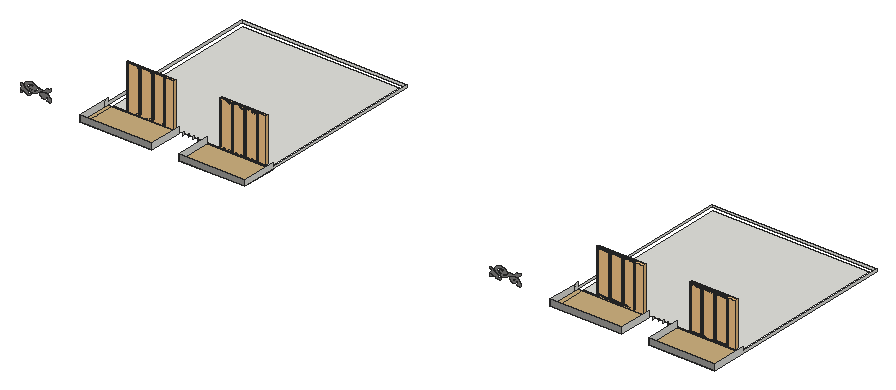
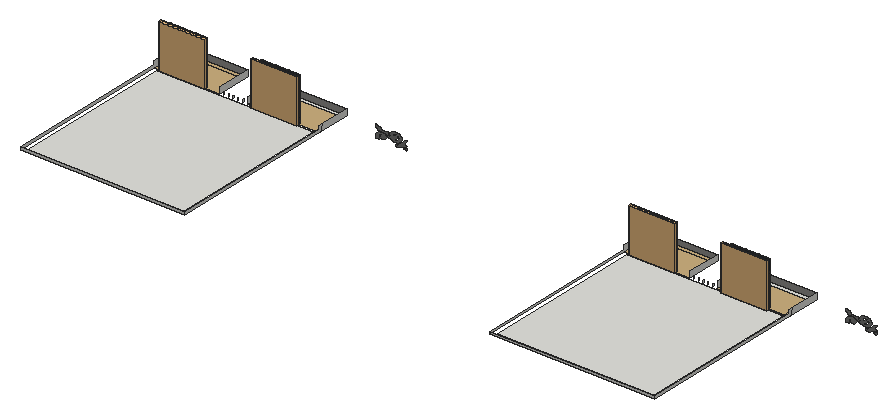
# SketchUp Ruby script. Lengths in inches.
U = 1.inch
M = Sketchup.active_model
def pt(a) = Geom::Point3d.new(a.map { |v| v * U })
def face(e, loops, mat)
  f = e.add_face(loops[0].map { |a| pt(a) })
  loops[1..].each { |l| e.add_face(l.map { |a| pt(a) }).erase! }
  f.material = f.back_material = mat if mat
  f
end
# faces: each face lists its corners as indices into pts; further lists are holes
def faces(e, pts, list, mat = nil) = list.each { |f| face(e, (f[0].is_a?(Array) ? f : [f]).map { |l| l.map { |i| pts[i] } }, mat) }
# xy, xz, yz: faces in a plane at the given z, y or x. An outline is a flat list of corners, or four numbers for a rectangle; further outlines are holes
def ring(l) = l.size == 4 ? [[l[0], l[1]], [l[2], l[1]], [l[2], l[3]], [l[0], l[3]]] : l.each_slice(2).to_a
def flat(e, list, mat, &to3) = list.each { |f| face(e, (f[0].is_a?(Array) ? f : [f]).map { |l| ring(l).map { |u, v| to3.(u, v) } }, mat) }
def xy(e, z, list, mat = nil) = flat(e, list, mat) { |x, y| [x, y, z] }
def xz(e, y, list, mat = nil) = flat(e, list, mat) { |x, z| [x, y, z] }
def yz(e, x, list, mat = nil) = flat(e, list, mat) { |y, z| [x, y, z] }
def lines(e, pts, list) = list.each { |a, b| e.add_line(pt(pts[a]), pt(pts[b])) }
# prism: a flat outline (further loops are holes) pulled along v
def prism(e, loops, v, mat = nil)
  f = face(e, loops, mat); d = Geom::Vector3d.new(v.map { |x| x * U })
  f.pushpull(f.normal.samedirection?(d) ? d.length : -d.length)
end
def box(e, o, s, mat = nil) = prism(e, [[o, [o[0] + s[0], o[1], o[2]], [o[0] + s[0], o[1] + s[1], o[2]], [o[0], o[1] + s[1], o[2]]]], [0, 0, s[2]], mat)
def at(x, y, z, deg = 0) = Geom::Transformation.translation(pt([x, y, z])) * Geom::Transformation.rotation(ORIGIN, Z_AXIS, deg.degrees)
def axes(o, x, y, z) = Geom::Transformation.new([*x, 0, *y, 0, *z, 0, *pt(o).to_a, 1])
def part(name) = M.definitions.add(name)
# library, detail: a bought-in or finely detailed component or shape, given as its bounding box
def library(name, o, s) = part(name).tap { |d| box(d.entities, o, s) }
def detail(e, o, s) = box(e.add_group.entities, o, s)
def put(e, d, t, mat = nil) = e.add_instance(d, t).tap { |i| i.material = mat if mat }
def group(e, t, mat = nil) = e.add_group.tap { |g| g.transformation = t; g.material = mat if mat }.entities
root = M.entities
M.materials.add("Wine2").color = [0, 0, 0]
M.materials["Wine2"].alpha = 0
M.materials.add("[0043_SaddleBrown]4").color = [124, 123, 122]
M.materials.add("[0130_Gainsboro]").color = [39, 45, 50]
M.materials.add("[Granite Light Gray]").color = [149, 148, 144]
M.materials.add("[Wood Floor Light]").color = [204, 176, 127]
c1 = part("Framed glazing panel")
xy(c1.entities,0,[[0,-0.98,43.07,0],[0,0,43.07,1.4]],"[0130_Gainsboro]")
xy(c1.entities,0.3,[[0.3,-1.43,42.77,-0.98]],"[0130_Gainsboro]")
xy(c1.entities,2.95,[[2.95,-1.43,40.12,-0.63],[2.95,-0.63,40.12,0],[2.95,0,40.12,0.64],[2.95,0.64,40.12,1.4]],"[0130_Gainsboro]")
xy(c1.entities,3.54,[[3.54,-0.63,39.53,0],[3.54,0,39.53,0.64]],"[0130_Gainsboro]")
xy(c1.entities,111.8125,[[3.54,-0.63,39.53,0],[3.54,0,39.53,0.64]],"[0130_Gainsboro]")
xy(c1.entities,112.4,[[2.95,-1.43,40.12,-0.63],[2.95,-0.63,40.12,0],[2.95,0,40.12,0.64],[2.95,0.64,40.12,1.4]],"[0130_Gainsboro]")
xy(c1.entities,115.05,[[0.3,-1.43,42.77,-0.98]],"[0130_Gainsboro]")
xy(c1.entities,115.35,[[0,-0.98,43.07,0],[0,0,43.07,1.4]],"[0130_Gainsboro]")
xz(c1.entities,-1.43,[[[0.3,0.3,42.77,115.05],[2.95,2.95,40.12,112.4]]],"[0130_Gainsboro]")
xz(c1.entities,-0.98,[[[0,0,43.07,115.35],[0.3,0.3,42.77,115.05]]],"[0130_Gainsboro]")
xz(c1.entities,-0.63,[[[2.95,2.95,40.12,112.4],[3.54,3.54,39.53,111.8125]]],"[0130_Gainsboro]")
xz(c1.entities,0,[[3.54,3.54,39.53,111.8125]],"Wine2")
xz(c1.entities,0,[[[0,0,43.07,115.35],[2.95,2.95,40.12,112.4]],[[2.95,2.95,40.12,112.4],[3.54,3.54,39.53,111.8125]]],"[0130_Gainsboro]")
xz(c1.entities,0.64,[[[2.95,2.95,40.12,112.4],[3.54,3.54,39.53,111.8125]]],"[0130_Gainsboro]")
xz(c1.entities,1.4,[[[0,0,43.07,115.35],[2.95,2.95,40.12,112.4]]],"[0130_Gainsboro]")
yz(c1.entities,0,[[-0.98,0,0,115.35],[0,0,1.4,115.35]],"[0130_Gainsboro]")
yz(c1.entities,0.3,[[-1.43,0.3,-0.98,115.05]],"[0130_Gainsboro]")
yz(c1.entities,2.95,[[-1.43,2.95,-0.63,112.4],[-0.63,2.95,0,112.4],[0,2.95,0.64,112.4],[0.64,2.95,1.4,112.4]],"[0130_Gainsboro]")
yz(c1.entities,3.54,[[-0.63,3.54,0,111.8125],[0,3.54,0.64,111.8125]],"[0130_Gainsboro]")
yz(c1.entities,39.53,[[-0.63,3.54,0,111.8125],[0,3.54,0.64,111.8125]],"[0130_Gainsboro]")
yz(c1.entities,40.12,[[-1.43,2.95,-0.63,112.4],[-0.63,2.95,0,112.4],[0,2.95,0.64,112.4],[0.64,2.95,1.4,112.4]],"[0130_Gainsboro]")
yz(c1.entities,42.77,[[-1.43,0.3,-0.98,115.05]],"[0130_Gainsboro]")
yz(c1.entities,43.07,[[-0.98,0,0,115.35],[0,0,1.4,115.35]],"[0130_Gainsboro]")
c2 = part("Glazing assembly")
put(c2.entities,c1,axes([90.57,1.43,0],[1.05148,0,0],[0,1,0],[0,0,1]))
put(c2.entities,c1,axes([0,1.43,0],[1.05148,0,0],[0,1,0],[0,0,1]))
put(c2.entities,c1,axes([45.29,1.43,0],[1.05148,0,0],[0,1,0],[0,0,1]))
c3 = library("Curtains",[0,0,0],[121.73,8.19,117.22])
xy(root,640.875,[[3103.26,651.03,3204.51,657.03],[3351.01,651.03,3452.26,657.03],[4353.89,651.03,4455.14,657.03],[4601.63,651.03,4702.88,657.03]])
xy(root,646.4375,[[3053.01,559.875,3243.69,570.83],[4303.63,559.875,4494.32,570.83],[3064.33,657.03,3480.11,1085.17],[4314.96,657.03,4730.74,1085.17]])
xy(root,646.4375,[[3316.14,559.875,3491.44,570.83],[4566.77,559.875,4742.06,570.83],[3053.01,570.83,3064.33,651.03],[3064.33,570.83,3243.69,651.03],[3316.14,570.83,3480.11,651.03],
  [3480.11,570.83,3491.44,651.03],[4303.63,570.83,4314.96,651.03],[4314.96,570.83,4494.32,651.03],[4566.77,570.83,4730.74,651.03],[4730.74,570.83,4742.06,651.03]],"[Wood Floor Light]")
xz(root,559.875,[[3053.01,646.4375,3243.69,662.4375],[3316.14,646.4375,3491.44,662.4375],[4303.63,646.4375,4494.32,662.4375],[4566.77,646.4375,4742.06,662.4375]],"[Granite Light Gray]")
xz(root,589.17,[[2869.93,640.49,2870.29,640.8,2870.68,641.09,2871.09,641.36,2871.54,641.62,2872.02,641.85,2872.52,642.07,2873.04,642.26,2873.59,642.43,2874.15,642.58,2874.73,642.71,2875.32,642.81,2875.92,642.89,2875.55,643.17,2875.15,643.4375,2874.72,643.68,2874.27,643.91,2873.79,644.125,2873.28,644.3125,2872.76,644.48,2872.22,644.62,2871.66,644.74,2871.1,644.83,2870.52,644.9,2869.93,644.94],[4120.56,640.49,4120.91,640.8,4121.3,641.09,4121.72,641.36,4122.17,641.62,4122.64,641.85,4123.15,642.07,4123.67,642.26,4124.21,642.43,4124.77,642.58,4125.35,642.71,4125.94,642.81,4126.54,642.89,4126.17,643.17,4125.78,643.4375,4125.35,643.68,4124.89,643.91,4124.41,644.125,4123.91,644.3125,4123.39,644.48,4122.85,644.62,4122.29,644.74,4121.72,644.83,4121.14,644.9,4120.56,644.94],[2893.58,641.03,2894.6,641.04,2895.41,641.12,2896.17,641.3125,2896.85,641.61,2897.4,641.99,2897.79,642.43,2898.01,642.92,2898.05,643.43,2897.9,643.93,2897.57,644.39,2897.08,644.8,2896.46,645.13,2895.73,645.37,2895.62,644.86,2895.3,644.38,2894.79,643.98,2894.125,643.66,2893.35,643.47,2892.52,643.4,2891.7,643.47,2890.92,643.66,2890.26,643.98,2889.75,644.38,2889.43,644.86,2889.32,645.37,2889.28,645.77,2889.25,646.18,2889.24,646.58,2889.25,646.99,2889.28,647.39,2889.32,647.8,2889.39,648.2,2889.47,648.6,2889.5625,649,2889.68,649.4,2889.8125,649.8,2889.96,650.19,2888.5,650.55,2887.09,650.99,2885.73,651.48,2884.45,652.05,2883.24,652.67,2882.12,653.35,2881.09,654.09,2880.16,654.87,2879.33,655.69,2878.62,656.56,2878.01,657.45,2877.52,658.375,2877,658.8,2876.45,659.22,2875.89,659.625,2875.3,660.02,2874.69,660.41,2874.06,660.78,2873.42,661.14,2872.76,661.49,2872.07,661.82,2871.375,662.14,2870.66,662.45,2869.93,662.74,2869.93,660.01,2870.95,659.23,2871.81,658.39,2872.49,657.48,2872.98,656.53,2873.28,655.56,2873.38,654.5625,2873.28,653.57,2872.98,652.59,2872.49,651.64,2871.81,650.74,2870.95,649.89,2869.93,649.12,2869.93,648.22,2871.22,648.05,2872.49,647.85,2873.74,647.6,2874.97,647.32,2876.18,647,2877.35,646.63,2878.49,646.23,2879.6,645.8,2880.67,645.33,2881.69,644.82,2882.67,644.28,2883.61,643.71,2884.34,643.28,2885.11,642.88,2885.94,642.51,2886.8,642.18,2887.7,641.89,2888.625,641.64,2889.58,641.43,2890.5625,641.26,2891.56,641.14,2892.57,641.0625],[4144.2,641.03,4145.22,641.04,4146.04,641.12,4146.8,641.3125,4147.47,641.61,4148.02,641.99,4148.42,642.43,4148.64,642.92,4148.68,643.43,4148.53,643.93,4148.2,644.39,4147.71,644.8,4147.08,645.13,4146.35,645.37,4146.24,644.86,4145.92,644.38,4145.41,643.98,4144.75,643.66,4143.98,643.47,4143.15,643.4,4142.32,643.47,4141.55,643.66,4140.88,643.98,4140.375,644.38,4140.06,644.86,4139.95,645.37,4139.9,645.77,4139.875,646.18,4139.87,646.58,4139.88,646.99,4139.9,647.39,4139.95,647.8,4140.01,648.2,4140.09,648.6,4140.1875,649,4140.3,649.4,4140.4375,649.8,4140.59,650.19,4139.125,650.55,4137.71,650.99,4136.36,651.48,4135.08,652.05,4133.87,652.67,4132.75,653.35,4131.72,654.09,4130.79,654.87,4129.96,655.69,4129.24,656.56,4128.64,657.45,4128.15,658.375,4127.625,658.8,4127.08,659.22,4126.51,659.625,4125.92,660.02,4125.32,660.41,4124.69,660.78,4124.04,661.14,4123.38,661.49,4122.7,661.82,4122,662.14,4121.29,662.45,4120.56,662.74,4120.56,660.01,4121.58,659.23,4122.43,658.39,4123.11,657.48,4123.61,656.53,4123.91,655.56,4124.01,654.5625,4123.91,653.57,4123.61,652.59,4123.11,651.64,4122.43,650.74,4121.58,649.89,4120.56,649.12,4120.56,648.22,4121.84,648.05,4123.12,647.85,4124.37,647.6,4125.6,647.32,4126.8,647,4127.98,646.63,4129.12,646.23,4130.22,645.8,4131.29,645.33,4132.32,644.82,4133.3,644.28,4134.23,643.71,4134.96,643.28,4135.74,642.88,4136.56,642.51,4137.42,642.18,4138.32,641.89,4139.25,641.64,4140.21,641.43,4141.1875,641.26,4142.18,641.14,4143.19,641.0625],[2950.32,642.71,2950.32,650.32,2949.96,650.87,2949.58,651.42,2949.18,651.96,2948.77,652.5,2948.35,653.03,2947.9,653.5625,2947.45,654.09,2946.97,654.61,2946.49,655.12,2945.99,655.63,2945.47,656.13,2944.94,656.63,2944.08,657.33,2943.1,657.96,2942,658.52,2940.8125,659,2939.54,659.39,2938.2,659.6875,2936.81,659.89,2935.39,659.99,2933.97,659.99,2932.56,659.89,2931.17,659.69,2929.83,659.39,2927.89,658.73,2926.2,657.86,2924.8125,656.81,2923.78,655.61,2923.15,654.31,2922.93,652.96,2923.15,651.61,2923.78,650.31,2924.8125,649.11,2926.2,648.05,2927.89,647.18,2929.83,646.53,2930.47,646.3,2931.16,646.13,2931.89,646.04,2932.63,646.01,2933.37,646.0625,2934.09,646.18,2934.77,646.37,2935.39,646.62,2935.93,646.93,2936.4,647.28,2936.76,647.68,2937.02,648.11,2937.38,648.49,2937.66,648.9,2937.83,649.33,2937.91,649.77,2937.88,650.21,2937.76,650.64,2937.54,651.0625,2937.22,651.46,2936.8125,651.82,2936.33,652.15,2935.77,652.43,2935.16,652.66,2934.8,652.54,2934.46,652.41,2934.13,652.27,2933.82,652.11,2933.53,651.94,2933.26,651.76,2933.01,651.57,2932.79,651.37,2932.58,651.15,2932.4,650.93,2932.25,650.71,2932.12,650.47,2931.35,650.76,2930.6875,651.12,2930.14,651.56,2929.74,652.05,2929.49,652.57,2929.41,653.12,2929.49,653.67,2929.74,654.19,2930.14,654.68,2930.6875,655.12,2931.35,655.48,2932.12,655.77,2933.05,655.79,2933.98,655.77,2934.91,655.7,2935.83,655.6,2936.73,655.45,2937.61,655.26,2938.47,655.03,2939.29,654.76,2940.09,654.46,2940.84,654.12,2941.55,653.75,2942.21,653.34,2942.79,652.56,2943.26,651.75,2943.61,650.91,2943.83,650.07,2943.93,649.21,2943.9,648.35,2943.75,647.49,2943.47,646.65,2943.07,645.82,2942.55,645.03,2941.92,644.26,2941.17,643.53,2941.93,643.69,2942.72,643.8125,2943.51,643.89,2944.32,643.93,2945.12,643.92,2945.92,643.87,2946.72,643.78,2947.49,643.64,2948.25,643.47,2948.97,643.25,2949.67,643],
  [4200.95,642.71,4200.95,650.32,4200.58,650.87,4200.2,651.42,4199.81,651.96,4199.4,652.5,4198.97,653.03,4198.53,653.5625,4198.07,654.09,4197.6,654.61,4197.11,655.12,4196.61,655.63,4196.1,656.13,4195.57,656.63,4194.71,657.33,4193.73,657.96,4192.63,658.52,4191.4375,659,4190.16,659.39,4188.82,659.6875,4187.43,659.89,4186.02,659.99,4184.6,659.99,4183.18,659.89,4181.79,659.69,4180.45,659.39,4178.52,658.73,4176.83,657.86,4175.4375,656.81,4174.41,655.61,4173.77,654.31,4173.56,652.96,4173.77,651.61,4174.41,650.31,4175.4375,649.11,4176.83,648.05,4178.52,647.18,4180.45,646.53,4181.1,646.3,4181.79,646.13,4182.51,646.04,4183.26,646.01,4184,646.0625,4184.71,646.18,4185.39,646.37,4186.01,646.62,4186.56,646.93,4187.02,647.28,4187.39,647.68,4187.64,648.11,4188.01,648.49,4188.28,648.9,4188.46,649.33,4188.53,649.77,4188.51,650.21,4188.38,650.64,4188.16,651.0625,4187.84,651.46,4187.4375,651.82,4186.95,652.15,4186.4,652.43,4185.78,652.66,4185.43,652.54,4185.09,652.41,4184.76,652.27,4184.45,652.11,4184.16,651.94,4183.89,651.76,4183.64,651.57,4183.41,651.37,4183.21,651.15,4183.03,650.93,4182.87,650.71,4182.74,650.47,4181.98,650.76,4181.3125,651.12,4180.77,651.56,4180.36,652.05,4180.12,652.57,4180.03,653.12,4180.12,653.67,4180.36,654.19,4180.77,654.68,4181.3125,655.12,4181.98,655.48,4182.74,655.77,4183.68,655.79,4184.61,655.77,4185.54,655.7,4186.45,655.6,4187.36,655.45,4188.24,655.26,4189.09,655.03,4189.92,654.76,4190.71,654.46,4191.46,654.12,4192.17,653.75,4192.83,653.34,4193.42,652.56,4193.89,651.75,4194.23,650.91,4194.46,650.07,4194.56,649.21,4194.53,648.35,4194.375,647.49,4194.1,646.65,4193.69,645.82,4193.17,645.03,4192.54,644.26,4191.8,643.53,4192.56,643.69,4193.34,643.8125,4194.14,643.89,4194.94,643.93,4195.75,643.92,4196.55,643.87,4197.34,643.78,4198.12,643.64,4198.87,643.47,4199.6,643.25,4200.29,643],[2900.61,650.01,2903.77,650.11,2906.85,650.55,2909.77,651.29,2912.44,652.33,2914.79,653.63,2916.75,655.16,2917.29,655.79,2917.88,656.41,2918.52,657.01,2919.2,657.59,2919.92,658.15,2920.69,658.6875,2921.5,659.2,2922.35,659.69,2923.23,660.16,2924.15,660.6,2925.1,661.01,2926.08,661.4,2927.38,661.78,2928.72,662.11,2930.08,662.4,2931.47,662.65,2932.875,662.84,2934.3,662.99,2935.73,663.09,2937.17,663.14,2938.61,663.14,2940.05,663.1,2941.48,663,2942.91,662.86,2943.46,663.4,2944.03,663.94,2944.61,664.48,2945.2,665.01,2945.8,665.54,2946.42,666.0625,2947.04,666.58,2948.32,667.6,2948.98,668.1,2949.65,668.59,2950.32,669.09,2950.32,674.83,2949.96,674.24,2949.46,673.68,2948.84,673.17,2948.11,672.72,2947.29,672.34,2946.38,672.04,2945.42,671.81,2944.41,671.67,2943.38,671.62,2942.35,671.65,2941.34,671.78,2940.37,671.99,2939.92,670.62,2939.11,669.32,2937.94,668.13,2936.47,667.08,2934.72,666.19,2932.75,665.51,2930.62,665.04,2928.38,664.8,2926.12,664.79,2923.89,665.03,2921.75,665.49,2919.78,666.17,2919.72,664.45,2919.25,662.75,2918.39,661.12,2917.14,659.57,2915.55,658.15,2913.64,656.89,2911.45,655.82,2909.04,654.95,2906.4375,654.3,2903.71,653.89,2900.92,653.73,2898.12,653.82,2895.67,654.4375,2893.45,655.33,2891.56,656.48,2890.07,657.82,2889.02,659.32,2888.47,660.91,2888.43,662.54,2888.89,664.14,2889.86,665.66,2891.28,667.03,2893.11,668.21,2895.27,669.15,2896.66,669.53,2898.16,669.73,2899.68,669.73,2901.18,669.55,2902.58,669.18,2903.83,668.64,2904.875,667.96,2905.67,667.16,2906.1875,666.28,2906.4,665.35,2906.3,664.42,2905.9,663.52,2905.62,663.1875,2905.24,662.89,2904.78,662.65,2904.25,662.48,2903.67,662.37,2903.06,662.33,2902.46,662.37,2901.88,662.48,2901.35,662.65,2900.89,662.89,2900.51,663.1875,2900.23,663.52,2900.09,663.71,2899.93,663.89,2899.75,664.07,2899.54,664.24,2899.31,664.39,2899.06,664.53,2898.79,664.66,2898.5,664.78,2898.2,664.88,2897.89,664.97,2897.57,665.04,2897.24,665.09,2896.66,664.88,2896.125,664.63,2895.64,664.34,2895.22,664.01,2894.87,663.66,2894.59,663.28,2894.39,662.89,2894.27,662.48,2894.23,662.07,2894.27,661.65,2894.4,661.25,2894.61,660.85,2895,660.32,2895.48,659.82,2896.04,659.36,2896.68,658.93,2897.4,658.55,2898.17,658.21,2899,657.94,2899.88,657.71,2900.79,657.55,2901.72,657.44,2902.66,657.4,2903.61,657.42,2905.1,657.57,2906.55,657.83,2907.92,658.22,2909.2,658.71,2910.37,659.3,2911.39,659.98,2912.26,660.74,2912.95,661.56,2913.46,662.4375,2913.78,663.35,2913.9,664.27,2913.81,665.2,2913.2,666.59,2912.28,667.91,2911.0625,669.15,2909.57,670.26,2907.84,671.23,2905.89,672.04,2903.79,672.67,2901.55,673.12,2899.24,673.36,2896.89,673.4,2894.5625,673.23,2892.29,672.86,2890.1,671.94,2888.12,670.85,2886.38,669.61,2884.92,668.25,2883.76,666.77,2882.92,665.22,2882.42,663.62,2882.26,661.99,2882.4375,660.36,2882.96,658.76,2883.82,657.21,2884.99,655.74,2886.8,654.15,2889.02,652.76,2891.59,651.63,2894.43,650.78,2897.46,650.23],[4151.23,650.01,4154.39,650.11,4157.47,650.55,4160.39,651.29,4163.07,652.33,4165.42,653.63,4167.375,655.16,4167.92,655.79,4168.51,656.41,4169.14,657.01,4169.82,657.59,4170.55,658.15,4171.32,658.6875,4172.125,659.2,4172.97,659.69,4173.85,660.16,4174.77,660.6,4175.72,661.01,4176.71,661.4,4178.01,661.78,4179.34,662.11,4180.71,662.4,4182.09,662.65,4183.5,662.84,4184.92,662.99,4186.35,663.09,4187.79,663.14,4189.24,663.14,4190.68,663.1,4192.11,663,4193.53,662.86,4194.09,663.4,4194.66,663.94,4195.24,664.48,4195.83,665.01,4196.43,665.54,4197.04,666.0625,4197.67,666.58,4198.3,667.09,4198.95,667.6,4199.6,668.1,4200.27,668.59,4200.95,669.09,4200.95,674.83,4200.58,674.24,4200.08,673.68,4199.46,673.17,4198.74,672.72,4197.91,672.34,4197.01,672.04,4196.04,671.81,4195.04,671.67,4194.01,671.62,4192.98,671.65,4191.97,671.78,4190.99,671.99,4190.55,670.62,4189.73,669.32,4188.57,668.13,4187.09,667.08,4185.34,666.19,4183.37,665.51,4181.24,665.04,4179.01,664.8,4176.74,664.79,4174.51,665.03,4172.38,665.49,4170.4,666.17,4170.34,664.45,4169.875,662.75,4169.01,661.12,4167.77,659.57,4166.18,658.15,4164.27,656.89,4162.08,655.82,4159.66,654.95,4157.0625,654.3,4154.34,653.89,4151.55,653.73,4148.75,653.82,4146.29,654.4375,4144.08,655.33,4142.19,656.48,4140.69,657.82,4139.65,659.32,4139.09,660.91,4139.05,662.54,4139.52,664.14,4140.48,665.66,4141.9,667.03,4143.73,668.21,4145.89,669.15,4147.29,669.53,4148.78,669.73,4150.31,669.73,4151.8,669.55,4153.2,669.18,4154.45,668.64,4155.5,667.96,4156.3,667.16,4156.8125,666.28,4157.03,665.35,4156.93,664.42,4156.52,663.52,4156.25,663.1875,4155.87,662.89,4155.4,662.65,4154.87,662.48,4154.29,662.37,4153.69,662.33,4153.09,662.37,4152.51,662.48,4151.97,662.65,4151.51,662.89,4151.13,663.1875,4150.86,663.52,4150.72,663.71,4150.56,663.89,4150.37,664.07,4150.16,664.24,4149.93,664.39,4149.68,664.53,4149.41,664.66,4149.13,664.78,4148.83,664.88,4148.52,664.97,4148.19,665.04,4147.86,665.09,4147.28,664.88,4146.75,664.63,4146.27,664.34,4145.85,664.01,4145.5,663.66,4145.22,663.28,4145.02,662.89,4144.9,662.48,4144.86,662.07,4144.9,661.65,4145.03,661.25,4145.23,660.85,4145.62,660.32,4146.1,659.82,4146.67,659.36,4147.31,658.93,4148.02,658.55,4148.8,658.21,4149.63,657.94,4150.5,657.71,4151.41,657.55,4152.34,657.44,4153.29,657.4,4154.23,657.42,4155.72,657.57,4157.17,657.83,4158.55,658.22,4159.83,658.71,4160.99,659.3,4162.02,659.98,4162.88,660.74,4163.58,661.56,4164.09,662.4375,4164.4,663.35,4164.52,664.27,4164.43,665.2,4163.83,666.59,4162.91,667.91,4161.6875,669.15,4160.19,670.26,4158.46,671.23,4156.52,672.04,4154.41,672.67,4152.18,673.12,4149.86,673.36,4147.52,673.4,4145.1875,673.23,4142.92,672.86,4140.72,671.94,4138.74,670.85,4137.01,669.61,4135.55,668.25,4134.39,666.77,4133.55,665.22,4133.04,663.62,4132.88,661.99,4133.0625,660.36,4133.59,658.76,4134.44,657.21,4135.62,655.74,4137.42,654.15,4139.64,652.76,4142.21,651.63,4145.05,650.78,4148.09,650.23]],"[0043_SaddleBrown]4")
xz(root,1096.5,[[3053.01,646.4375,3491.44,652.4375],[4303.63,646.4375,4742.06,652.4375]])
yz(root,3053.01,[[559.875,646.4375,640.11,662.4375],[640.11,646.4375,640.11,662.4375,651.03,662.4375,651.03,652.4375,1096.5,652.4375,1096.5,646.4375]])
yz(root,3243.69,[[559.875,646.4375,647.91,662.4375]])
yz(root,3256.69,[[647.91,646.4375,651.03,652.4375]])
yz(root,3269.44,[[648.85,646.4375,651.03,652.4375]])
yz(root,3281.57,[[648.85,646.4375,651.03,652.4375]])
yz(root,3293.94,[[648.85,646.4375,651.03,652.4375]])
yz(root,3306.82,[[648.85,646.4375,651.03,652.4375]])
yz(root,3316.14,[[559.875,646.4375,651.03,662.4375]])
yz(root,3491.44,[[559.875,646.4375,1096.5,646.4375,1096.5,652.4375,651.03,652.4375,651.03,662.4375,559.875,662.4375]])
yz(root,4303.63,[[559.875,646.4375,640.11,662.4375],[640.11,646.4375,640.11,662.4375,651.03,662.4375,651.03,652.4375,1096.5,652.4375,1096.5,646.4375]])
yz(root,4494.32,[[559.875,646.4375,647.91,662.4375]])
yz(root,4507.32,[[647.91,646.4375,651.03,652.4375]])
yz(root,4520.07,[[648.85,646.4375,651.03,652.4375]])
yz(root,4532.19,[[648.85,646.4375,651.03,652.4375]])
yz(root,4544.57,[[648.85,646.4375,651.03,652.4375]])
yz(root,4557.44,[[648.85,646.4375,651.03,652.4375]])
yz(root,4566.77,[[559.875,646.4375,651.03,662.4375]])
yz(root,4742.06,[[559.875,646.4375,1096.5,646.4375,1096.5,652.4375,651.03,652.4375,651.03,662.4375,559.875,662.4375]])
put(root,c2,axes([3103.26,651.74,649.48],[0.75,0,0],[0,0.75,0],[0,0,1.01765]))
put(root,c3,at(3105.59,651.74,646.65))
put(root,c2,axes([3350.36,651.03,649.48],[0.75,0,0],[0,0.75,0],[0,0,1.01765]))
put(root,c3,at(3351.01,651.03,649.66))
put(root,c2,axes([4353.89,651.74,649.48],[0.75,0,0],[0,0.75,0],[0,0,1.01765]))
put(root,c3,at(4356.22,651.74,646.65))
put(root,c2,axes([4600.98,651.03,649.48],[0.75,0,0],[0,0.75,0],[0,0,1.01765]))
put(root,c3,at(4601.63,651.03,649.66))
